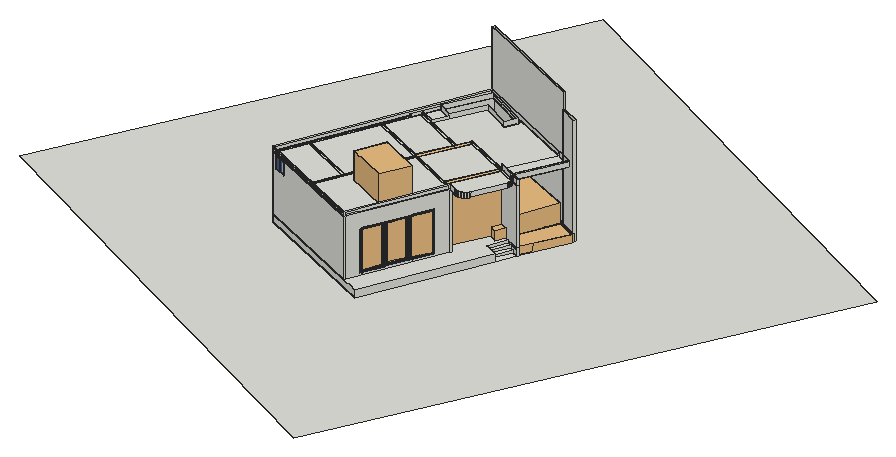
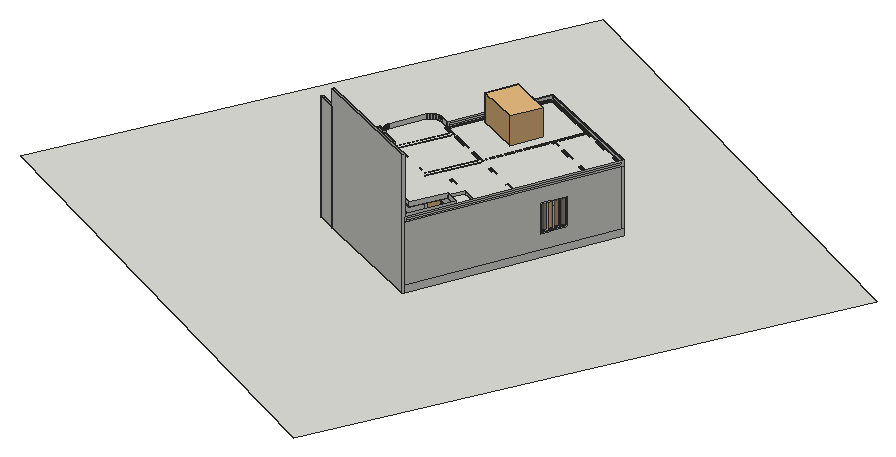
# SketchUp Ruby script. Lengths in inches.
U = 1.inch
M = Sketchup.active_model
def pt(a) = Geom::Point3d.new(a.map { |v| v * U })
def face(e, loops, mat)
  f = e.add_face(loops[0].map { |a| pt(a) })
  loops[1..].each { |l| e.add_face(l.map { |a| pt(a) }).erase! }
  f.material = f.back_material = mat if mat
  f
end
# faces: each face lists its corners as indices into pts; further lists are holes
def faces(e, pts, list, mat = nil) = list.each { |f| face(e, (f[0].is_a?(Array) ? f : [f]).map { |l| l.map { |i| pts[i] } }, mat) }
# xy, xz, yz: faces in a plane at the given z, y or x. An outline is a flat list of corners, or four numbers for a rectangle; further outlines are holes
def ring(l) = l.size == 4 ? [[l[0], l[1]], [l[2], l[1]], [l[2], l[3]], [l[0], l[3]]] : l.each_slice(2).to_a
def flat(e, list, mat, &to3) = list.each { |f| face(e, (f[0].is_a?(Array) ? f : [f]).map { |l| ring(l).map { |u, v| to3.(u, v) } }, mat) }
def xy(e, z, list, mat = nil) = flat(e, list, mat) { |x, y| [x, y, z] }
def xz(e, y, list, mat = nil) = flat(e, list, mat) { |x, z| [x, y, z] }
def yz(e, x, list, mat = nil) = flat(e, list, mat) { |y, z| [x, y, z] }
def lines(e, pts, list) = list.each { |a, b| e.add_line(pt(pts[a]), pt(pts[b])) }
# prism: a flat outline (further loops are holes) pulled along v
def prism(e, loops, v, mat = nil)
  f = face(e, loops, mat); d = Geom::Vector3d.new(v.map { |x| x * U })
  f.pushpull(f.normal.samedirection?(d) ? d.length : -d.length)
end
def box(e, o, s, mat = nil) = prism(e, [[o, [o[0] + s[0], o[1], o[2]], [o[0] + s[0], o[1] + s[1], o[2]], [o[0], o[1] + s[1], o[2]]]], [0, 0, s[2]], mat)
def at(x, y, z, deg = 0) = Geom::Transformation.translation(pt([x, y, z])) * Geom::Transformation.rotation(ORIGIN, Z_AXIS, deg.degrees)
def axes(o, x, y, z) = Geom::Transformation.new([*x, 0, *y, 0, *z, 0, *pt(o).to_a, 1])
def part(name) = M.definitions.add(name)
# library, detail: a bought-in or finely detailed component or shape, given as its bounding box
def library(name, o, s) = part(name).tap { |d| box(d.entities, o, s) }
def detail(e, o, s) = box(e.add_group.entities, o, s)
def put(e, d, t, mat = nil) = e.add_instance(d, t).tap { |i| i.material = mat if mat }
def group(e, t, mat = nil) = e.add_group.tap { |g| g.transformation = t; g.material = mat if mat }.entities
root = M.entities
M.materials.add("Wine2").color = [0, 0, 0]
M.materials["Wine2"].alpha = 0
M.materials.add("[0130_Gainsboro]").color = [39, 45, 50]
M.materials.add("[Translucent Glass Blue]").color = [100, 149, 237]
M.materials["[Translucent Glass Blue]"].alpha = 0.5
M.materials.add("[Translucent_Glass_Gray]4").color = [128, 128, 128]
M.materials["[Translucent_Glass_Gray]4"].alpha = 0.5
c1 = library("Group\#75",[0,0,0],[122.08,51.81,18.73])
c2 = library("Sectional sofa",[-0.93,-10.63,-23.92],[126.92,88.46,78.25])
c3 = library("KOŁO+DRZWI+WNĘKOWE+SKRZYDŁOWE+NEXT+80,+PRAWOSTRONNE+HDRF80R\#",[0.43,0.44,0],[31.07,2.7,98.875])
c4 = library("porta 4",[0.2,-5.42,1.33],[46.55,4.72,83.21])
c5 = library("KOŁO+DRZWI+WNĘKOWE+SKRZYDŁOWE+NEXT+80,+PRAWOSTRONNE+HDRF80R",[-3.72,0,0],[35.22,3.14,98.875])
c6 = library("Group8\#1",[-48.75,-20.06,-0.03],[97.5,40.12,31.8])
c7 = library("Group\#46",[0,0,0],[59.88,84.57,74.8])
c8 = library("Kohler_Balast_1935.skp\#1",[-38.83,-18.45,0],[74.81,42.21,2.86])
c9 = part("Group\#12")
box(c9.entities,[0,0,0],[5,144,144])
c10 = library("Bedroom furniture set",[0,-4.61,0],[113.04,95.21,114.59])
c11 = library("Group\#66",[0,0,0],[120.1,9.95,144])
c12 = library("Dining table set",[0,0,0],[65.45,109.33,43.4])
c13 = library("3d flower - flower pot",[-12.2,-15.73,0],[29.88,29.15,27.8])
c14 = part("Group\#4")
prism(c14.entities,[[[0,298,0],[0,-5,0],[0,-5,144],[0,298,144]],[[0,39.33,108],[0,39.33,139.52],[0,7,139.52],[0,7,108]]],[5,0,0])
c15 = part("Group\#11")
prism(c15.entities,[[[0,149,0],[0,41.99,0],[0,41.99,78],[0,2.99,78],[0,2.99,0],[0,-149,0],[0,-149,144],[0,149,144]]],[5,0,0])
c16 = library("Group13\#1",[-103.57,-19.82,-0.03],[42.43,40.67,31.4])
c17 = part("Group\#117")
xy(c17.entities,0,[[0,0,36,10]])
g1 = group(c17.entities,at(-0.41,0,0))
g2 = group(g1,at(0,0,0))
xy(g2,6,[[0.41,0,36.41,10]])
xz(g2,0,[[0.41,0,36.41,6]])
xz(g2,10,[[0.41,0,36.41,6]])
yz(g2,0.41,[[0,0,10,6]])
yz(g2,36.41,[[0,0,10,6]])
c18 = library("CC18",[-599.2,17.07,4.47],[949.25,1548.15,446.11])
c19 = part("Group\#74")
xy(c19.entities,0,[[0,-0.98,43.07,0],[0,0,43.07,1.4]],"[0130_Gainsboro]")
xy(c19.entities,0.3,[[0.3,-1.43,42.77,-0.98]],"[0130_Gainsboro]")
xy(c19.entities,2.95,[[2.95,-1.43,40.12,-0.63],[2.95,-0.63,40.12,0],[2.95,0,40.12,0.64],[2.95,0.64,40.12,1.4]],"[0130_Gainsboro]")
xy(c19.entities,3.54,[[3.54,-0.63,39.53,0],[3.54,0,39.53,0.64]],"[0130_Gainsboro]")
xy(c19.entities,111.8125,[[3.54,-0.63,39.53,0],[3.54,0,39.53,0.64]],"[0130_Gainsboro]")
xy(c19.entities,112.4,[[2.95,-1.43,40.12,-0.63],[2.95,-0.63,40.12,0],[2.95,0,40.12,0.64],[2.95,0.64,40.12,1.4]],"[0130_Gainsboro]")
xy(c19.entities,115.05,[[0.3,-1.43,42.77,-0.98]],"[0130_Gainsboro]")
xy(c19.entities,115.35,[[0,-0.98,43.07,0],[0,0,43.07,1.4]],"[0130_Gainsboro]")
xz(c19.entities,-1.43,[[[0.3,0.3,42.77,115.05],[2.95,2.95,40.12,112.4]]],"[0130_Gainsboro]")
xz(c19.entities,-0.98,[[[0,0,43.07,115.35],[0.3,0.3,42.77,115.05]]],"[0130_Gainsboro]")
xz(c19.entities,-0.63,[[[2.95,2.95,40.12,112.4],[3.54,3.54,39.53,111.8125]]],"[0130_Gainsboro]")
xz(c19.entities,0,[[3.54,3.54,39.53,111.8125]],"Wine2")
xz(c19.entities,0,[[[0,0,43.07,115.35],[2.95,2.95,40.12,112.4]],[[2.95,2.95,40.12,112.4],[3.54,3.54,39.53,111.8125]]],"[0130_Gainsboro]")
xz(c19.entities,0.64,[[[2.95,2.95,40.12,112.4],[3.54,3.54,39.53,111.8125]]],"[0130_Gainsboro]")
xz(c19.entities,1.4,[[[0,0,43.07,115.35],[2.95,2.95,40.12,112.4]]],"[0130_Gainsboro]")
yz(c19.entities,0,[[-0.98,0,0,115.35],[0,0,1.4,115.35]],"[0130_Gainsboro]")
yz(c19.entities,0.3,[[-1.43,0.3,-0.98,115.05]],"[0130_Gainsboro]")
yz(c19.entities,2.95,[[-1.43,2.95,-0.63,112.4],[-0.63,2.95,0,112.4],[0,2.95,0.64,112.4],[0.64,2.95,1.4,112.4]],"[0130_Gainsboro]")
yz(c19.entities,3.54,[[-0.63,3.54,0,111.8125],[0,3.54,0.64,111.8125]],"[0130_Gainsboro]")
yz(c19.entities,39.53,[[-0.63,3.54,0,111.8125],[0,3.54,0.64,111.8125]],"[0130_Gainsboro]")
yz(c19.entities,40.12,[[-1.43,2.95,-0.63,112.4],[-0.63,2.95,0,112.4],[0,2.95,0.64,112.4],[0.64,2.95,1.4,112.4]],"[0130_Gainsboro]")
yz(c19.entities,42.77,[[-1.43,0.3,-0.98,115.05]],"[0130_Gainsboro]")
yz(c19.entities,43.07,[[-0.98,0,0,115.35],[0,0,1.4,115.35]],"[0130_Gainsboro]")
c20 = part("Glazed door assembly")
put(c20.entities,c19,axes([90.57,1.43,0],[1.05148,0,0],[0,1,0],[0,0,1]))
put(c20.entities,c19,axes([0,1.43,0],[1.05148,0,0],[0,1,0],[0,0,1]))
put(c20.entities,c19,axes([45.29,1.43,0],[1.05148,0,0],[0,1,0],[0,0,1]))
c21 = library("Group14",[-64.97,9.24,0.31],[138.52,9.93,292.57])
c22 = library("Group16",[86.37,-10.76,76.46],[21.79,14.87,35.97])
c23 = library("Group22",[48.82,-10.91,0.23],[97.72,18.57,293.12])
c24 = library("Group24",[44.03,2.01,0.26],[103.73,11,292.35])
c25 = library("Group27",[-106.21,-10.76,76.46],[21.8,14.87,35.97])
c26 = library("Group35",[-145.81,2.01,0.26],[103.73,11,292.35])
c27 = library("Group33",[-144.59,-10.91,0.23],[97.72,18.57,293.12])
c28 = part("Group\#71")
put(c28.entities,c21,at(145.81,10.91,-0.23))
put(c28.entities,c22,at(145.81,10.91,-0.23))
put(c28.entities,c23,at(145.81,10.91,-0.23))
put(c28.entities,c24,at(145.81,10.91,-0.23))
put(c28.entities,c25,at(145.81,10.91,-0.23))
put(c28.entities,c26,at(145.81,10.91,-0.23))
put(c28.entities,c27,at(145.81,10.91,-0.23))
c29 = library("bathroom kit",[-10.19,-11.89,-0.14],[22.08,39.51,30.77])
c30 = library("Shower_03.skp",[-9.2,-8.46,-0.03],[13.92,58.47,24.25])
c31 = part("Component\#36")
prism(c31.entities,[[[0,70.87,0],[0,0,0],[0,0,47.24],[0,70.87,47.24]],[[0,1.97,1.97],[0,68.9,1.97],[0,68.9,45.28],[0,1.97,45.28]]],[7.875,0,0])
c32 = part("Component\#34")
xy(c32.entities,0,[[0,0,3.9375,16.73]])
xy(c32.entities,0.98,[[0,0.98,1.77,15.75],[1.77,0.98,2.85,15.75],[2.85,0.98,3.9375,15.75]])
xy(c32.entities,42.32,[[0,0.98,1.77,15.75],[1.77,0.98,2.85,15.75],[2.85,0.98,3.9375,15.75]])
xy(c32.entities,43.31,[[0,0,3.9375,16.73]])
xz(c32.entities,0,[[0,0,3.9375,43.31]])
xz(c32.entities,0.98,[[0,0.98,1.77,42.32],[1.77,0.98,2.85,42.32],[2.85,0.98,3.9375,42.32]])
xz(c32.entities,15.75,[[0,0.98,1.77,42.32],[1.77,0.98,2.85,42.32],[2.85,0.98,3.9375,42.32]])
xz(c32.entities,16.73,[[0,0,3.9375,43.31]])
yz(c32.entities,0,[[[0,0,16.73,43.31],[0.98,0.98,15.75,42.32]]])
yz(c32.entities,1.77,[[0.98,0.98,15.75,42.32]],"[Translucent_Glass_Gray]4")
yz(c32.entities,2.85,[[0.98,0.98,15.75,42.32]],"[Translucent_Glass_Gray]4")
yz(c32.entities,3.9375,[[[0,0,16.73,43.31],[0.98,0.98,15.75,42.32]]])
c33 = part("simple window")
p = [[0,68.9,1.97],[0,35.43,1.97]]
lines(c33.entities,p,[[0,1]])
put(c33.entities,c31,at(0,0,0))
put(c33.entities,c32,axes([1.14,52.17,1.97],[0.71,0,0],[0,1,0],[0,0,1]))
put(c33.entities,c32,axes([1.14,1.97,1.97],[0.71,0,0],[0,1,0],[0,0,1]))
put(c33.entities,c32,axes([3.9375,18.7,1.97],[0.71,0,0],[0,1,0],[0,0,1]))
put(c33.entities,c32,axes([3.9375,35.43,1.97],[0.71,0,0],[0,1,0],[0,0,1]))
c34 = part("Group\#67")
xy(c34.entities,0,[[0,0,36,10]])
g3 = group(c34.entities,at(-0.41,0,0))
g4 = group(g3,at(0,0,0))
xy(g4,6,[[0.41,0,36.41,35.24]])
xz(g4,0,[[0.41,0,36.41,6]])
xz(g4,35.24,[[0.41,0,36.41,6]])
yz(g4,0.41,[[0,0,35.24,6]])
yz(g4,36.41,[[0,0,35.24,6]])
c35 = part("Group\#53")
xy(c35.entities,0,[[0,0,36,10]])
g5 = group(c35.entities,at(-0.41,0,0))
g6 = group(g5,at(0,0,0))
xy(g6,6,[[0.41,0,36.41,10]])
xz(g6,0,[[0.41,0,36.41,6]])
xz(g6,10,[[0.41,0,36.41,6]])
yz(g6,0.41,[[0,0,10,6]])
yz(g6,36.41,[[0,0,10,6]])
c36 = part("Janela aluminio")
xy(c36.entities,0,[[0,0,47.24,1.57],[23.62,1.57,47.24,2.76],[0,2.76,25.98,3.9375],[0,3.9375,47.24,5.91]])
xy(c36.entities,43.31,[[0,0,47.24,1.57],[23.62,1.57,47.24,2.76],[0,2.76,0,5.91,47.24,5.91,47.24,3.9375,25.98,3.9375,25.98,2.76],[25.98,2.76,47.24,3.9375]])
xz(c36.entities,1.57,[[0,0,23.62,0,23.62,41.34,21.26,41.34,21.26,1.97,1.97,1.97,1.97,41.34,23.62,41.34,23.62,43.31,0,43.31],[[23.62,0,47.24,43.31],[25.7,1.97,45.28,41.34]]])
xz(c36.entities,2.76,[[[0,0,23.62,43.31],[2.36,2.36,21.26,40.94]],[23.62,0,25.98,43.31]])
xz(c36.entities,2.76,[[2.36,2.36,21.26,40.94]],"[Translucent Glass Blue]")
xz(c36.entities,3.9375,[[25.98,0,25.98,2.36,44.88,2.36,44.88,40.94,25.98,40.94,25.98,43.31,47.24,43.31,47.24,0]])
xz(c36.entities,3.9375,[[25.98,2.36,44.88,40.94]],"[Translucent Glass Blue]")
yz(c36.entities,0,[[0,0,1.57,43.31],[2.76,0,5.91,43.31]])
yz(c36.entities,23.62,[[1.57,0,2.76,43.31]])
yz(c36.entities,25.98,[[2.76,0,3.9375,43.31]])
yz(c36.entities,47.24,[[0,0,1.57,43.31],[1.57,0,2.76,43.31],[3.9375,0,5.91,43.31]])
xy(root,-12,[[1080.487,974.318,1037.378,995.251,1037.567,995.168,1039.564,999.752,1082.673,978.819],[1037.567,995.168,1037.378,995.251,1039.564,999.752],[1037.378,995.251,759.771,1116.157,761.767,1120.741,1039.564,999.752],[759.771,1116.157,761.767,1120.741,759.581,1116.239],[759.581,1116.239,761.767,1120.741,761.578,1120.823]])
xy(root,6,[[841.72,546.009,837.135,548.006,930.972,763.458,935.556,761.462]])
xy(root,12,[[854.098,574.43,921.181,728.456,916.597,730.453,849.514,576.427]])
xy(root,114,[[854.098,574.43,849.514,576.427,916.597,730.453,921.181,728.456]])
xy(root,150,[[[839.724,541.426,561.938,662.44,759.581,1116.239,1020.479,1002.61,965.832,890.07,1008.199,869.498,1008.321,869.75,1008.56,870.241,1008.777,870.687,1009.049,871.248,1031.219,861.592,1031.281,861.565,1029.287,856.98,1013.436,863.883,1015.41,862.5,1017.591,860.436,1019.447,858.074,1020.938,855.466,1022.032,852.669,1022.704,849.741,1022.942,846.747,1022.739,843.75,1022.099,840.815,1021.052,838.042,988.203,762.502,986.785,759.762,985.014,757.237,982.92,754.972,980.541,753.008,977.921,751.38,975.106,750.118,972.148,749.245,969.099,748.775,966.015,748.719,964.937,748.845,962.951,749.076,960.919,749.596,959.962,749.841,957.103,750.999,935.556,761.462,930.972,763.458,837.135,548.006,841.717,546.01],[754.403,984.89,791.688,1061.675,861.065,1027.987,874.577,1055.816,805.201,1089.503,769.05,1106.497,718.473,1002.337],[687.595,943.915,699.209,967.833,698.513,968.171],[769.05,1106.497,769.27,1106.95,764.512,1109.261,764.263,1108.747,764.272,1108.743],[764.263,1108.747,762.284,1109.708,762.244,1109.626]],[841.72,546.009,934.755,759.624,934.632,759.678,841.717,546.01],[841.717,546.01,837.135,548.006,930.972,763.458,935.556,761.462,934.755,759.624,934.632,759.678],[1031.472,861.482,1031.283,861.564,1031.286,861.572],[1031.283,861.564,1031.281,861.565,1031.285,861.573,1031.286,861.572],
  [1031.281,861.565,1031.219,861.592,1031.224,861.602,1031.285,861.573],[1008.199,869.498,965.832,890.07,972.0625,887.356,1008.321,869.75],[1008.321,869.75,972.0625,887.356,984.197,882.071,1008.56,870.241],[1008.56,870.241,984.197,882.071,995.208,877.276,1008.777,870.687],[1008.777,870.687,995.208,877.276,1009.049,871.248],
  [1009.049,871.248,995.208,877.276,984.197,882.071,972.0625,887.356,965.832,890.07,1020.479,1002.61,1062.846,982.038],[687.595,943.915,698.513,968.171,699.209,967.833],[805.201,1089.503,769.05,1106.497,769.27,1106.95],[769.05,1106.497,764.272,1108.743,764.263,1108.747,764.512,1109.261,769.27,1106.95],[764.263,1108.747,762.244,1109.626,762.284,1109.708]])
xy(root,150.652,[[1011.161,868.784,1008.484,870.084,1008.56,870.241,1011.238,868.941],[1011.238,868.941,1008.56,870.241,1008.777,870.687,1011.454,869.387],[1011.454,869.387,1008.777,870.687,1009.049,871.248,1011.726,869.947],[1011.726,869.947,1009.049,871.248,1062.561,981.452,1065.239,980.152]])
xy(root,161.348,[[1011.161,868.784,1011.238,868.941,1008.56,870.241,1008.484,870.084],[1011.238,868.941,1011.454,869.387,1008.777,870.687,1008.56,870.241],[1011.454,869.387,1011.726,869.947,1009.049,871.248,1008.777,870.687],[1011.726,869.947,1065.239,980.152,1062.561,981.452,1009.049,871.248]])
p = [[1037.378,995.251,264.897],[1037.378,995.251,-12],[1080.487,974.318,-12],[1080.487,974.318,264.897],[1082.673,978.819,-12],[1082.673,978.819,264.897],
  [1039.564,999.752,-12],[1039.564,999.752,264.897],[1020.479,1002.61,162],[1020.479,1002.61,150],[759.581,1116.239,150],[759.581,1116.239,-12],
  [759.771,1116.157,-12],[1037.378,995.251,306],[781.771,1106.575,306],[759.581,1116.239,306],[759.581,1116.239,162],[764.166,1114.243,162],
  [761.767,1120.741,-12],[761.767,1120.741,306],[1039.374,999.835,306],[1039.564,999.752,306],[1030.348,860.141,0.027],[1030.355,860.139,-0.05],
  [1030.674,860,-0.017],[1030.667,860.003,0.06],[1030.029,860.296,0.072],[1030.036,860.293,-0.006],[1030.355,860.154,0.027],[1030.348,860.157,0.105],
  [1029.71,860.451,0.117],[1029.717,860.448,0.039],[1030.035,860.309,0.072],[1030.029,860.312,0.15],[1029.391,860.605,0.161],[1029.398,860.602,0.084],
  [1029.716,860.464,0.117],[1029.71,860.467,0.194],[1029.072,860.76,0.206],[1029.079,860.757,0.128],[1029.397,860.618,0.161],[1029.391,860.621,0.239],
  [1028.746,860.902,0.25],[1028.753,860.899,0.173],[1029.065,860.763,0.283],[1028.421,861.043,0.295],[1028.428,861.04,0.217],[1028.74,860.905,0.328],
  [1028.102,861.198,0.339],[1028.109,861.195,0.262],[1028.427,861.056,0.295],[1028.421,861.059,0.372],[1027.783,861.353,0.384],[1027.79,861.35,0.306],
  [1028.108,861.211,0.339],[1028.102,861.214,0.417],[1027.464,861.507,0.429],[1027.471,861.504,0.351],[1027.789,861.366,0.384],[1027.782,861.368,0.462],
  [1027.145,861.662,0.473],[1027.151,861.659,0.396],[1027.47,861.52,0.429],[1027.463,861.523,0.506],[1026.826,861.816,0.518],[1026.832,861.813,0.44],
  [1027.151,861.675,0.473],[1027.144,861.678,0.551],[1026.506,861.971,0.5625],[1026.513,861.968,0.485],[1026.832,861.829,0.518],[1026.825,861.832,0.595],
  [1026.1875,862.126,0.607],[1026.194,862.123,0.529],[1026.513,861.984,0.5625],[1026.506,861.987,0.64],[1025.868,862.28,0.651],[1025.875,862.277,0.574],
  [1026.194,862.139,0.607],[1026.187,862.142,0.684],[1025.549,862.435,0.696],[1025.556,862.432,0.619],[1025.875,862.293,0.652],[1025.868,862.296,0.729],
  [1025.23,862.59,0.741],[1025.237,862.587,0.663],[1025.555,862.448,0.696],[1025.549,862.451,0.774],[1024.911,862.744,0.785],[1024.918,862.741,0.708],
  [1025.236,862.603,0.741],[1025.23,862.605,0.818],[1024.592,862.899,0.83],[1024.599,862.896,0.752],[1024.917,862.757,0.785],[1024.911,862.76,0.863],
  [1024.266,863.04,0.874],[1024.273,863.038,0.797],[1024.585,862.902,0.907],[1023.941,863.182,0.919],[1023.948,863.179,0.841],[1024.26,863.043,0.952],
  [1023.622,863.337,0.963],[1023.629,863.334,0.886],[1023.947,863.195,0.919],[1023.941,863.198,0.996],[1023.303,863.491,1.008],[1023.31,863.488,0.93],
  [1023.628,863.35,0.963],[1023.622,863.353,1.041],[1022.984,863.646,1.053],[1022.991,863.643,0.975],[1023.309,863.504,1.008],[1023.302,863.507,1.086],
  [1022.665,863.801,1.097],[1022.671,863.798,1.02],[1022.99,863.659,1.053],[1022.983,863.662,1.13],[1022.346,863.955,1.142],[1022.352,863.952,1.064],
  [1022.671,863.814,1.097],[1022.664,863.817,1.175],[1022.026,864.11,1.186],[1022.033,864.107,1.109],[1022.352,863.968,1.142],[1022.345,863.971,1.219],
  [1021.707,864.265,1.231],[1021.714,864.262,1.153],[1022.033,864.123,1.186],[1022.026,864.126,1.264],[1021.388,864.419,1.275],[1021.395,864.416,1.198],
  [1021.714,864.277,1.231],[1021.707,864.28,1.309],[1021.069,864.574,1.32],[1021.076,864.571,1.243],[1021.395,864.432,1.276],[1021.388,864.435,1.353],
  [1020.75,864.728,1.365],[1020.757,864.725,1.287],[1021.075,864.587,1.32],[1021.069,864.59,1.398],[1020.431,864.883,1.409],[1020.4375,864.88,1.332],
  [1020.756,864.741,1.365],[1020.75,864.744,1.442],[1020.112,865.038,1.454],[1020.119,865.035,1.376],[1020.437,864.896,1.409],[1020.43,864.899,1.487],
  [1019.786,865.179,1.498],[1019.793,865.176,1.421],[1020.105,865.041,1.531],[1019.461,865.321,1.543],[1019.468,865.318,1.465],[1019.78,865.182,1.576],
  [1019.142,865.476,1.587],[1019.149,865.473,1.51],[1019.467,865.334,1.543],[1019.461,865.337,1.62],[1018.823,865.63,1.632],[1018.83,865.627,1.555],
  [1019.148,865.489,1.588],[1019.141,865.491,1.665],[1018.504,865.785,1.677],[1018.511,865.782,1.599],[1018.829,865.643,1.632],[1018.822,865.646,1.71],
  [1018.185,865.939,1.721],[1018.191,865.937,1.644],[1018.51,865.798,1.677],[1018.503,865.801,1.754],[1017.866,866.094,1.766],[1017.872,866.091,1.688],
  [1018.191,865.952,1.721],[1018.184,865.955,1.799],[1017.546,866.249,1.81],[1017.553,866.246,1.733],[1017.872,866.107,1.766],[1017.865,866.11,1.843],
  [1017.227,866.403,1.855],[1017.234,866.4,1.777],[1017.553,866.262,1.81],[1017.546,866.265,1.888],[1016.908,866.558,1.9],[1016.915,866.555,1.822],
  [1017.234,866.416,1.855],[1017.227,866.419,1.933],[1016.589,866.713,1.944],[1016.596,866.71,1.867],[1016.915,866.571,1.9],[1016.908,866.574,1.977],
  [1016.27,866.867,1.989],[1016.277,866.864,1.911],[1016.595,866.726,1.944],[1016.589,866.728,2.022],[1015.951,867.022,2.033],[1015.958,867.019,1.956],
  [1016.276,866.88,1.989],[1016.27,866.883,2.066],[1015.632,867.176,2.078],[1015.639,867.174,2],[1015.957,867.035,2.033],[1015.95,867.038,2.111],
  [1015.306,867.318,2.122],[1015.313,867.315,2.045],[1015.625,867.179,2.155],[837.135,548.006,6],[841.72,546.009,6],[841.72,546.009,150],
  [841.717,546.01,150],[837.135,548.006,150],[935.556,761.462,6],[935.556,761.462,150],[934.755,759.624,150],[854.098,574.43,12],
  [854.098,574.43,114],[921.181,728.456,114],[921.181,728.456,12],[930.972,763.458,150],[930.972,763.458,6],[916.597,730.453,12],
  [916.597,730.453,114],[849.514,576.427,114],[849.514,576.427,12],[1008.321,869.75,147.996],[1008.56,870.241,147.996],[1008.777,870.687,147.996],
  [1009.049,871.248,147.996],[1063.721,983.841,147.996],[1063.721,983.841,164.004],[1009.049,871.248,164.004],[1008.777,870.687,164.004],[1008.56,870.241,164.004],
  [1008.321,869.75,164.004],[1007.324,867.695,164.004],[1007.324,867.695,147.996],[1008.321,869.75,150],[1008.199,869.498,150],[1008.199,869.498,162],
  [1008.321,869.75,162],[1008.56,870.241,162],[1008.777,870.687,162],[1009.049,871.248,162],[1062.846,982.038,162],[1062.846,982.038,150],
  [1009.049,871.248,150],[1008.777,870.687,150],[1008.56,870.241,150],[561.938,662.44,150],[839.724,541.426,150],[839.724,541.426,162],
  [561.938,662.44,162],[564.5625,661.297,159.138],[837.1,542.57,159.138],[837.1,542.57,152.862],[564.5625,661.297,152.862],[934.632,759.678,150],
  [934.632,759.678,162],[841.717,546.01,162],[841.717,546.01,159.138],[933.491,757.053,159.138],[933.491,757.053,152.862],[841.717,546.01,152.862],
  [840.865,544.051,152.862],[840.865,544.051,159.138],[758.439,1113.615,159.138],[563.081,665.064,159.138],[563.081,665.064,152.862],[758.439,1113.615,152.862],
  [966.015,748.719,162],[964.937,748.845,162],[964.937,748.845,150],[966.015,748.719,150],[969.099,748.775,162],[969.099,748.775,150],
  [962.951,749.076,162],[962.951,749.076,150],[972.148,749.245,162],[972.148,749.245,150],[960.919,749.596,162],[960.919,749.596,150],
  [975.106,750.118,162],[975.106,750.118,150],[959.962,749.841,162],[959.962,749.841,150],[957.103,750.999,162],[957.103,750.999,150],
  [977.921,751.38,162],[977.921,751.38,150],[935.556,761.462,162],[980.541,753.008,162],[980.541,753.008,150],[982.92,754.972,162],
  [982.92,754.972,150],[985.014,757.237,162],[985.014,757.237,150],[986.785,759.762,162],[986.785,759.762,150],[934.755,759.624,162],
  [988.203,762.502,162],[988.203,762.502,150],[1021.036,838.006,162],[1021.052,838.042,150],[1021.052,838.042,162],[1022.099,840.815,162],
  [1022.099,840.815,150],[1022.739,843.75,162],[1022.739,843.75,150],[1022.942,846.747,162],[1022.942,846.747,150],[1022.704,849.741,162],
  [1022.704,849.741,150],[1022.032,852.669,162],[1022.032,852.669,150],[1020.938,855.466,162],[1020.938,855.466,150],[1019.447,858.074,162],
  [1019.447,858.074,150],[1031.472,861.482,162],[1029.476,856.897,162],[1029.476,856.897,150],[1031.472,861.482,150],[1029.287,856.98,162],
  [1013.436,863.883,162],[1013.436,863.883,150],[1029.287,856.98,150],[1017.591,860.436,162],[1017.591,860.436,150],[1015.41,862.5,162],
  [1015.41,862.5,150],[1031.283,861.564,150],[1031.281,861.565,150],[1031.219,861.592,150],[995.208,877.276,150],[984.197,882.071,150],
  [972.0625,887.356,150],[965.832,890.07,150],[965.832,890.07,162],[972.0625,887.356,162],[984.197,882.071,162],[995.208,877.276,162],
  [1028.364,862.835,162],[1031.219,861.592,162],[1031.281,861.565,162],[1031.283,861.564,162],[1009.049,871.248,150.652],[1008.777,870.687,150.652],
  [1008.56,870.241,150.652],[1008.484,870.084,150.652],[1008.484,870.084,161.348],[1008.56,870.241,161.348],[1008.777,870.687,161.348],[1009.049,871.248,161.348],
  [1062.561,981.452,161.348],[1062.561,981.452,150.652],[689.576,942.953,150],[689.576,942.953,156],[687.595,943.915,156],[687.595,943.915,150],
  [687.569,943.857,150],[687.569,943.857,156],[698.513,968.171,150],[698.513,968.171,156],[737.892,950.886,150],[701.189,966.871,150],
  [701.189,966.871,156],[737.892,950.886,156],[754.403,984.89,156],[754.403,984.89,150],[699.209,967.833,150],[761.416,1107.922,156],
  [761.416,1107.922,150],[718.473,1002.337,150],[718.473,1002.337,162],[754.403,984.89,162],[791.688,1061.675,162],[791.688,1061.675,150],
  [769.05,1106.497,150],[769.05,1106.497,156],[769.05,1106.497,162],[861.065,1027.987,162],[861.065,1027.987,150],[874.577,1055.816,150],
  [874.577,1055.816,162],[874.577,1055.816,156],[805.201,1089.503,156],[805.201,1089.503,150],[764.272,1108.743,150],[764.272,1108.743,156],
  [762.284,1109.708,156],[762.244,1109.626,150],[762.284,1109.708,150],[764.263,1108.747,156],[764.263,1108.747,150],[1011.161,868.784,150.652],
  [1011.161,868.784,161.348],[1011.454,869.387,150.652],[1011.726,869.947,150.652],[1065.239,980.152,150.652],[1065.239,980.152,161.348],[1011.726,869.947,161.348],
  [1011.454,869.387,161.348],[1011.238,868.941,161.348],[1011.238,868.941,150.652],[805.201,1089.503,162],[751.923,1100.529,150],[764.512,1109.261,156],
  [764.512,1109.261,150],[762.169,1109.659,150]]
faces(root,p,[[0,1,2,3],[2,4,5,3],[6,7,5,4],[8,9,10,11,12,1,0,13,14,15,16,17],[7,6,1,0],[6,18,19,20,21,7],[18,11,10,16,15,19],[22,23,24,25],
  [26,27,28,29],[30,31,32,33],[34,35,36,37],[38,39,40,41],[42,43,38,44],[45,46,42,47],[48,49,50,51],[52,53,54,55],
  [56,57,58,59],[60,61,62,63],[64,65,66,67],[68,69,70,71],[72,73,74,75],[76,77,78,79],[80,81,82,83],[84,85,86,87],
  [88,89,90,91],[92,93,94,95],[96,97,92,98],[99,100,96,101],[102,103,104,105],[106,107,108,109],[110,111,112,113],[114,115,116,117],
  [118,119,120,121],[122,123,124,125],[126,127,128,129],[130,131,132,133],[134,135,136,137],[138,139,140,141],[142,143,144,145],[146,147,148,149],
  [150,151,146,152],[153,154,150,155],[156,157,158,159],[160,161,162,163],[164,165,166,167],[168,169,170,171],[172,173,174,175],[176,177,178,179],
  [180,181,182,183],[184,185,186,187],[188,189,190,191],[192,193,194,195],[196,197,198,199],[200,201,202,203],[204,205,200,206],[207,208,209,210,211],
  [[209,208,212,213,214],[215,216,217,218]],[[219,220,207,211],[221,222,223,224]],[212,220,219,213],[215,224,223,216],[217,222,221,218],[[225,226,227,228,229,230,231,232,233,234,235,236],[237,238,239,240,241,242,243,244,245,246,247,248]],[[249,250,251,252],[253,254,255,256]],[[210,257,258,259,251,250],[260,261,262,263,264,265]],
  [[10,249,252,16],[266,267,268,269]],[270,271,272,273],[274,270,273,275],[271,276,277,272],[278,274,275,279],[276,280,281,277],[282,278,279,283],[280,284,285,281],
  [284,286,287,285],[288,282,283,289],[286,290,213,287],[291,288,289,292],[293,291,292,294],[295,293,294,296],[297,295,296,298],[257,214,299,258],
  [290,299,214,213],[300,297,298,301],[302,300,301,303,304],[305,304,303,306],[307,305,306,308],[309,307,308,310],[311,309,310,312],[313,311,312,314],
  [315,313,314,316],[317,315,316,318],[319,320,321,322],[323,324,325,326],[327,317,318,328],[329,327,328,330],[319,322,331,332,333,246,334,335,336,337,338,339,340,341,243,342,343,344,345],[324,329,330,325],
  [338,337,238,239],[[238,237,248,247,246,245,244,243,242,241,240,239],[346,347,348,349,350,351,352,353,354,355]],[356,357,358,359],[357,356,360,361],[360,359,358,361],[359,362,363,358],[364,365,366,367],[367,368,369,364],
  [365,370,362,363,366],[371,363,362,372],[9,8,244,245],[369,373,374,375,368],[375,376,377,369,368],[373,378,379,380,374],[17,8,9,10,16],[377,376,381,382],
  [383,382,381,384,385],[386,387,383,385],[386,379,378,387],[388,378,379,389],[390,371,372,391,392],[393,390,392,394],[393,394,388,389],[350,349,395,396],
  [397,398,399,400,401,402,403,396,395,404],[355,354,400,399],[254,253,256,255],[261,260,265,264,263,262],[267,266,269,268],[405,386,385,384],[380,379,386,405]])
lines(root,p,[[10,406],[407,408],[409,391]])
put(root,c1,axes([1028.97,858.28,-10.9],[0.4537,0.9361,-0.00956],[-0.89085,0.43163,-0.01363],[-0.00838,0.01427,0.99986]))
put(root,c1,axes([1029.01,858.35,-11.44],[0.43614,0.89987,-0.00472],[-0.89982,0.43605,-0.01377],[-0.01034,0.01025,0.99989]))
put(root,c2,axes([787.93,731.87,8.13],[0.78284,-0.34527,0],[-0.34527,-0.78284,0],[0,0,0.8556]))
g7 = group(root,at(865.03,960.15,0,-113.535))
xy(g7,-12,[[-101,-159,-101,144,24,144,24,192,29,192,29,176,77,176,77,192,393.97,192,393.97,-159],[29,176,77,192]])
xy(g7,-6,[[29,166,77,176]])
xy(g7,0,[[29,156,77,166]])
xy(g7,6,[[-101,-159,393.97,-159,393.97,192,77,192,77,156,29,156,29,192,24,192,24,144,-101,144]])
xz(g7,-159,[[-101,-12,393.97,6]])
xz(g7,144,[[-101,-12,24,6]])
xz(g7,156,[[29,0,77,6]])
xz(g7,166,[[29,-6,77,0]])
xz(g7,176,[[29,-12,77,-6]])
xz(g7,192,[[24,-12,29,6],[77,-12,393.97,6]])
yz(g7,-101,[[-159,-12,144,6]])
yz(g7,24,[[144,-12,192,6]])
yz(g7,29,[[176,-12,192,-12,192,0,166,0,166,-6,176,-6],[156,0,192,6]])
yz(g7,77,[[176,-12,176,-6,166,-6,166,0,192,0,192,-12],[156,0,192,6]])
yz(g7,393.97,[[-159,-12,192,6]])
p = [[24,144,6],[29,144,6]]
lines(g7,p,[[0,1]])
g8 = group(root,at(1143.86,0,-12,64.1))
xy(g8,0,[[0,0,1290.49,1271.58]])
put(root,c3,axes([680.21,652.39,5.99],[-1.10532,0.49586,0],[0.40931,0.9124,0],[0,0,1]))
put(root,c3,axes([681.01,655.04,5.99],[1.10532,-0.49586,0],[-0.40931,-0.9124,0],[0,0,1]))
put(root,c4,axes([837.12,803.24,4.74],[-0.76347,0.34639,0],[-0.41316,-0.91066,0],[0,0,0.93759]))
put(root,c4,axes([827.14,905.64,4.74],[-0.55696,0.25269,0],[-0.41316,-0.91066,0],[0,0,0.93749]))
put(root,c5,axes([646.6,668.76,6],[0.48304,1.08503,0],[-0.91356,0.4067,0],[0,0,1]))
put(root,c6,axes([922.57,854,6.02],[-0.37135,-0.85264,0],[0.91682,-0.3993,0],[0,0,0.79]))
put(root,c7,at(664.81,885.02,6,-23.435))
put(root,c8,axes([687.53,674.23,6],[-0.91179,0.41065,0],[-0.36093,-0.80138,0],[0,0,1]))
put(root,c9,at(599.32,735.6,6,-113.535))
put(root,c10,at(601.37,738.72,6,-23.1))
put(root,c11,at(844.55,937.65,6,-115.9))
put(root,c11,at(959.15,887.74,6,-115.9))
put(root,c12,axes([901.1875,706.89,6],[0.34729,0.84112,0],[-0.84112,0.34729,0],[0,0,0.91]))
put(root,c13,axes([968.74,869.03,6],[0.35381,0.72864,0],[-0.72864,0.35381,0],[0,0,0.81]))
put(root,c14,at(568.52,665.03,6,-113.535))
put(root,c15,at(800.95,825.54,6,-113.535))
g9 = group(root,at(846.27,942.14,6,-113.535))
box(g9,[0,0,0],[5,202,144])
g10 = group(root,at(705.02,605.32,6,64.1))
xy(g10,0,[[0.21,0,0,5,3.03,5.12,3.23,0.125],[34.8,1.43,34.59,6.42,192.84,12.96,193.04,7.97],[193.04,7.97,232.01,9.58,231.8,14.57,192.84,12.96],[232.01,9.58,231.8,14.57,234.8,14.69,235.01,9.7]])
xy(g10,78,[[3.23,0.125,3.03,5.12,34.59,6.42,34.8,1.43]])
xy(g10,79.24,[[193.04,7.97,192.84,12.96,231.8,14.57,232.01,9.58]])
xy(g10,144,[[0.21,0,3.23,0.125,235.01,9.7,234.8,14.69,0,5]])
p = [[0,5,0],[0.21,0,0],[0.21,0,144],[0,5,144],[3.23,0.125,0],[3.23,0.125,78],
  [3.23,0.125,144],[3.03,5.12,0],[3.03,5.12,78],[235.01,9.7,144],[34.8,1.43,78],[34.8,1.43,0],
  [193.04,7.97,0],[193.04,7.97,79.24],[232.01,9.58,79.24],[232.01,9.58,0],[235.01,9.7,0],[34.59,6.42,78],
  [34.59,6.42,0],[234.8,14.69,0],[231.8,14.57,0],[231.8,14.57,79.24],[192.84,12.96,79.24],[192.84,12.96,0],
  [234.8,14.69,144]]
faces(g10,p,[[0,1,2,3],[4,5,6,2,1],[5,4,7,8],[9,6,5,10,11,12,13,14,15,16],[11,10,17,18],[19,20,21,22,23,18,17,8,7,0,3,24],[13,12,23,22],[15,14,21,20],
  [16,19,24,9]])
g11 = group(root,at(717.26,1019.06,6,-113.535))
prism(g11,[[[-106,0,0],[384,0,0],[384,0,144],[-106,0,144]],[[203.27,0,108],[263.27,0,108],[263.27,0,36],[203.27,0,36]]],[0,5,0])
put(root,c16,at(892.48,973.34,6.03,64.1))
put(root,c17,at(795.4,925.84,6,66.285))
g12 = group(root,at(701.375,966.79,6))
prism(g12,[[[-2.83,-4.22,0],[99.99,-49,0],[99.99,-49,77.95],[126.07,-60.36,77.95],[126.07,-60.36,0],[128.82,-61.56,0],[128.82,-61.56,144],[-2.83,-4.22,144]]],[2,4.58,0])
put(root,c18,axes([862.66,995.28,5.54],[-0.03848,-0.09429,0],[0.09429,-0.03848,0],[0,0,0.10184]))
put(root,c4,axes([719.37,637.2,4.76],[-0.27098,-0.6222,0],[0.91682,-0.3993,0],[0,0,0.93749]))
put(root,c4,axes([798.2,818.2,6],[-0.33455,-0.76814,0],[0.91682,-0.3993,0],[0,0,0.93749]))
put(root,c20,axes([854.07,574.36,11.73],[0.49513,1.13686,0],[-0.91682,0.3993,0],[0,0,0.89]))
put(root,c28,axes([846.74,575.16,12],[0.25356,0.52218,0],[-0.45877,0.22277,0],[0,0,0.3672]))
put(root,c17,at(786.25,929.86,12,66.285))
put(root,c29,at(618.6,710.1,13.64,-115.9))
put(root,c17,at(777.09,933.88,18,66.285))
put(root,c17,at(767.9375,937.9,24,66.285))
put(root,c17,at(758.78,941.93,30,66.285))
put(root,c17,at(749.625,945.95,36,66.285))
put(root,c30,axes([721.72,656.52,45.85],[-0.37601,-0.92662,0],[0,0,1],[-0.92662,0.37601,0]))
put(root,c33,axes([612.13,777.68,42],[0.91682,-0.3993,0],[0.34739,0.79763,0],[0,0,1.524]))
put(root,c17,at(740.47,949.97,42,66.285))
put(root,c34,at(731.3125,953.99,48,66.285))
put(root,c17,at(749.8125,996.11,54,156.285))
put(root,c17,at(753.84,1005.26,60,156.285))
put(root,c17,at(757.86,1014.42,66,156.285))
put(root,c17,at(761.88,1023.57,72,156.285))
put(root,c17,at(765.9,1032.73,78,156.285))
put(root,c35,at(769.92,1041.89,84,156.285))
g13 = group(root,at(769.92,1041.89,90,66.285))
xy(g13,0,[[0,0,36,10]])
g14 = group(g13,at(-0.41,0,0))
g15 = group(g14,at(0,0,0))
xy(g15,6,[[0.41,0,61.41,35.24]])
xz(g15,0,[[0.41,0,61.41,6]])
xz(g15,35.24,[[0.41,0,61.41,6]])
yz(g15,0.41,[[0,0,35.24,6]])
yz(g15,61.41,[[0,0,35.24,6]])
put(root,c17,at(788.375,1059.03,96,66.285))
put(root,c17,at(797.53,1055,102,66.285))
put(root,c17,at(806.6875,1050.98,108,66.285))
put(root,c36,axes([603.27,647.43,114],[-0.62484,0.2578,0],[-0.1373,-0.33279,0],[0,0,0.72049]))
put(root,c17,at(815.84,1046.96,114,66.285))
put(root,c17,at(825,1042.9375,120,66.285))
put(root,c17,at(834.15,1038.92,126,66.285))
put(root,c17,at(843.31,1034.89,132,66.285))
put(root,c17,at(852.46,1030.87,138,66.285))
put(root,c17,at(861.62,1026.85,144,66.285))
put(root,c2,axes([787.93,731.87,170.13],[0.78284,-0.34527,0],[-0.34527,-0.78284,0],[0,0,0.8556]))
